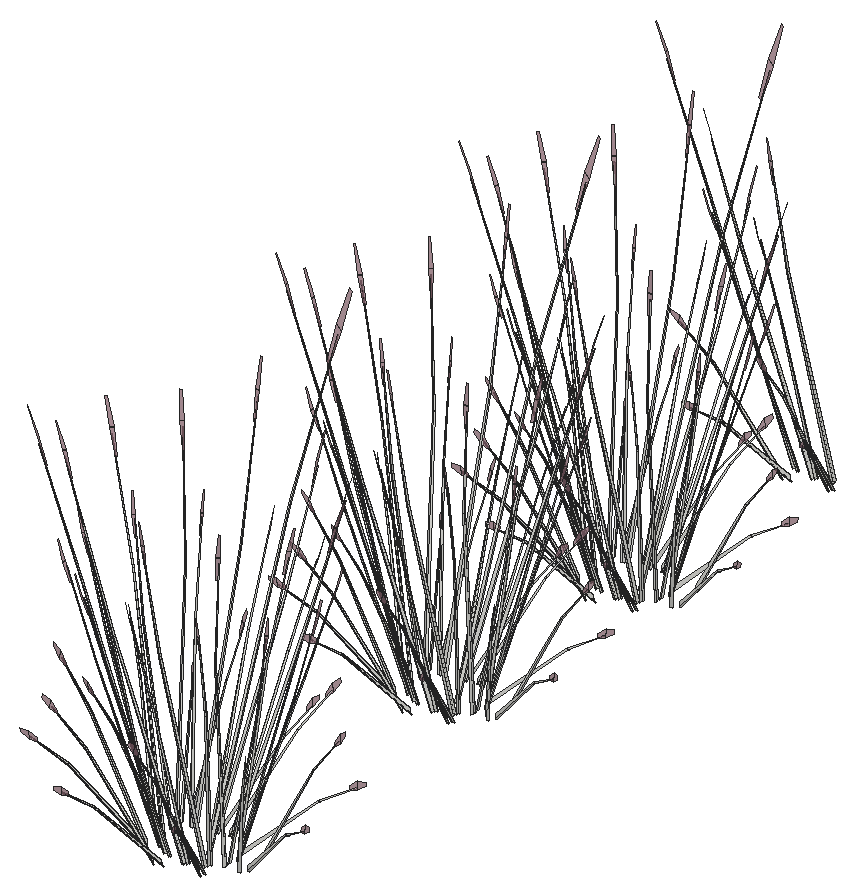
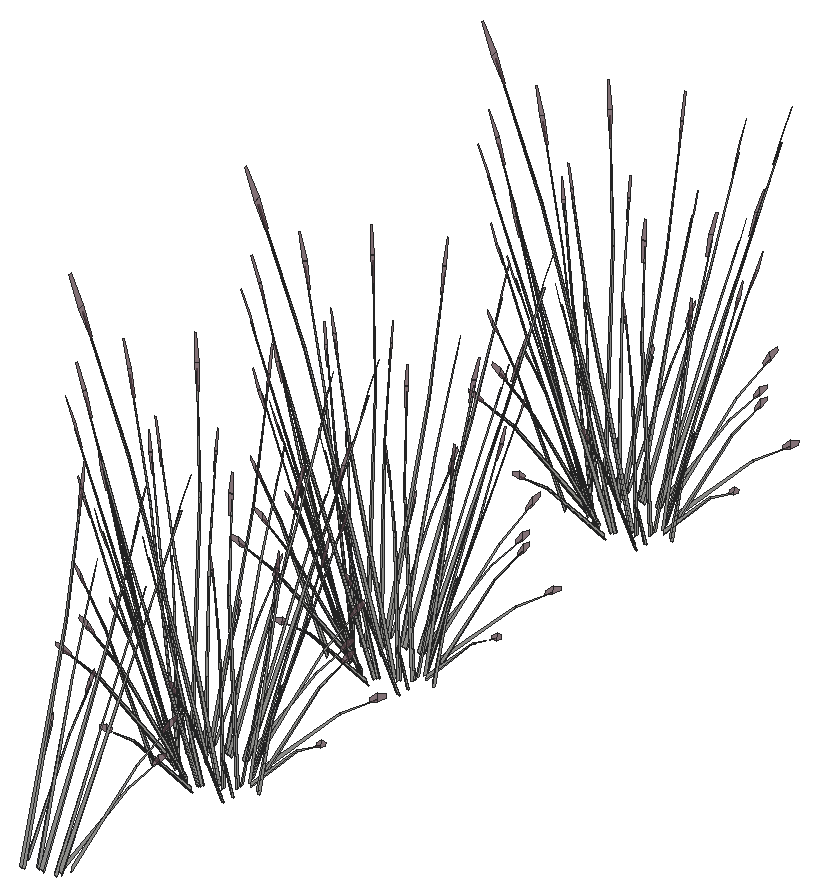
# SketchUp Ruby script. Lengths in inches.
U = 1.inch
M = Sketchup.active_model
def pt(a) = Geom::Point3d.new(a.map { |v| v * U })
def face(e, loops, mat)
  f = e.add_face(loops[0].map { |a| pt(a) })
  loops[1..].each { |l| e.add_face(l.map { |a| pt(a) }).erase! }
  f.material = f.back_material = mat if mat
  f
end
# faces: each face lists its corners as indices into pts; further lists are holes
def faces(e, pts, list, mat = nil) = list.each { |f| face(e, (f[0].is_a?(Array) ? f : [f]).map { |l| l.map { |i| pts[i] } }, mat) }
# xy, xz, yz: faces in a plane at the given z, y or x. An outline is a flat list of corners, or four numbers for a rectangle; further outlines are holes
def ring(l) = l.size == 4 ? [[l[0], l[1]], [l[2], l[1]], [l[2], l[3]], [l[0], l[3]]] : l.each_slice(2).to_a
def flat(e, list, mat, &to3) = list.each { |f| face(e, (f[0].is_a?(Array) ? f : [f]).map { |l| ring(l).map { |u, v| to3.(u, v) } }, mat) }
def xy(e, z, list, mat = nil) = flat(e, list, mat) { |x, y| [x, y, z] }
def xz(e, y, list, mat = nil) = flat(e, list, mat) { |x, z| [x, y, z] }
def yz(e, x, list, mat = nil) = flat(e, list, mat) { |y, z| [x, y, z] }
def lines(e, pts, list) = list.each { |a, b| e.add_line(pt(pts[a]), pt(pts[b])) }
# prism: a flat outline (further loops are holes) pulled along v
def prism(e, loops, v, mat = nil)
  f = face(e, loops, mat); d = Geom::Vector3d.new(v.map { |x| x * U })
  f.pushpull(f.normal.samedirection?(d) ? d.length : -d.length)
end
def box(e, o, s, mat = nil) = prism(e, [[o, [o[0] + s[0], o[1], o[2]], [o[0] + s[0], o[1] + s[1], o[2]], [o[0], o[1] + s[1], o[2]]]], [0, 0, s[2]], mat)
def at(x, y, z, deg = 0) = Geom::Transformation.translation(pt([x, y, z])) * Geom::Transformation.rotation(ORIGIN, Z_AXIS, deg.degrees)
def axes(o, x, y, z) = Geom::Transformation.new([*x, 0, *y, 0, *z, 0, *pt(o).to_a, 1])
def part(name) = M.definitions.add(name)
# library, detail: a bought-in or finely detailed component or shape, given as its bounding box
def library(name, o, s) = part(name).tap { |d| box(d.entities, o, s) }
def detail(e, o, s) = box(e.add_group.entities, o, s)
def put(e, d, t, mat = nil) = e.add_instance(d, t).tap { |i| i.material = mat if mat }
def group(e, t, mat = nil) = e.add_group.tap { |g| g.transformation = t; g.material = mat if mat }.entities
root = M.entities
M.materials.add("LightPink_Translucent").color = [144, 107, 117]
M.materials["LightPink_Translucent"].alpha = 0.75
c1 = part("blade")
p = [[2.15,0.21,22],[0,0.17,0],[0.09,0.45,0],[2.18,0.31,22],[2.29,0.31,22],[0.38,0.45,0],
  [2.48,0.24,33],[2.49,0.24,33],[2.48,0.22,33]]
faces(c1.entities,p,[[0,1,2,3],[4,5,2,3],[6,3,4,7],[8,0,3,6]])
c2 = part("seeds")
p = [[0.3,-0.1,1.38],[-0.01,-0.03,1.59],[-0.01,-0.03,0.03],[0.14,-0.07,-0.07],[0.29,-0.03,3],[0.15,0.01,3.11]]
faces(c2.entities,p,[[0,1,2,3],[1,0,4,5]],"LightPink_Translucent")
c3 = part("blade with seeds")
put(c3.entities,c1,at(0,0,0))
put(c3.entities,c2,axes([2.4,0.25,30.99],[1.5799,-0.05474,1.17369],[-0.12525,1.92788,0.29478],[-0.07173,-0.02425,1.56792]))
put(root,c3,axes([671.4,165.1,513.91],[-0.09951,-0.08005,1.45204],[-0.66407,0.05075,-0.22964],[-0.10598,-0.19148,0.11645]))
put(root,c3,axes([674.39,166.08,513.91],[-0.00628,-0.11364,1.45204],[-0.53042,-0.32843,-0.22964],[0.08201,-0.19909,0.11645]))
put(root,c3,axes([674.24,165.68,513.91],[-0.06607,0.04361,1.47228],[-0.64734,-0.14714,-0.13912],[-0.02343,-0.19032,0.26054]))
put(root,c3,axes([670.72,164.84,513.91],[-0.01214,0.06844,1.47228],[-0.59861,0.24837,-0.13912],[-0.17615,-0.12696,0.26054]))
put(root,c3,axes([672.41,166.34,514.18],[-0.63664,0.26583,-0.10093],[-0.31286,-0.47181,-0.56021],[-0.084,-0.19882,0.85122]))
put(root,c3,axes([673.74,166.9375,514.18],[-0.71502,-0.02829,-0.10093],[0.01954,-0.53563,-0.56021],[0.04967,-0.20629,0.85122]))
put(root,c3,axes([672.4,166.125,513.93],[0.47939,-0.19405,0.05337],[0.23464,0.35385,0.42015],[-0.0463,-0.15598,0.64067]))
put(root,c3,axes([670.76,166.18,513.93],[0.29569,-0.36271,0.05337],[0.42107,0.21117,0.42015],[-0.13613,-0.11629,0.64067]))
put(root,c3,axes([670.89,166.14,514.51],[-0.4342,0.54737,-0.11304],[-0.6288,-0.31535,-0.62743],[-0.21858,-0.15465,0.95337]))
put(root,c3,axes([673.85,166.75,513.93],[0.53464,0.0266,0.05337],[-0.01466,0.40172,0.42015],[0.05594,-0.15388,0.64067]))
put(root,c3,axes([669.22,165.98,513.91],[-0.13998,-0.00403,1.45204],[-0.44565,0.40302,-0.22964],[-0.23779,-0.08235,0.11645]))
put(root,c3,axes([674.51,167.99,514.18],[-0.60181,-0.31483,-0.10093],[0.34671,-0.45593,-0.56021],[0.17003,-0.15849,0.85122]))
put(root,c3,axes([675.99,167.85,513.91],[-0.08498,-0.00434,1.47228],[-0.35287,-0.46464,-0.13912],[0.14171,-0.15278,0.26054]))
put(root,c3,axes([669.37,166.89,513.93],[0.03276,-0.43418,0.05337],[0.49468,0.0119,0.42015],[-0.18949,-0.04543,0.64067]))
put(root,c3,axes([674.73,167.875,513.93],[0.44663,0.24013,0.05337],[-0.26003,0.34195,0.42015],[0.14319,-0.11055,0.64067]))
put(root,c3,axes([676.32,168.41,513.91],[0.09028,-0.08697,1.45204],[-0.11555,-0.53348,-0.22964],[0.22652,-0.10115,0.11645]))
put(root,c3,axes([668.6875,166.33,513.91],[0.04823,0.05698,1.47228],[-0.23252,0.51221,-0.13912],[-0.23548,0.00371,0.26054]))
put(root,c3,axes([669.6,166.99,514.18],[-0.03484,0.58066,-0.10093],[-0.65957,-0.01587,-0.56021],[-0.25402,-0.04034,0.85122]))
put(root,c3,axes([674.54,169.22,514.18],[-0.32734,-0.51701,-0.10093],[0.58097,-0.25407,-0.56021],[0.24483,-0.06821,0.85122]))
put(root,c3,axes([668.6,168.08,513.93],[-0.23895,-0.38931,0.05337],[0.43573,-0.19055,0.42015],[-0.19208,0.0376,0.64067]))
put(root,c3,axes([674.8,169.21,513.93],[0.23895,0.38931,0.05337],[-0.43573,0.19055,0.42015],[0.19208,-0.0376,0.64067]))
put(root,c3,axes([675.84,170.75,513.91],[-0.05883,-0.04999,1.47228],[0.12868,-0.53581,-0.13912],[0.23172,-0.03423,0.26054]))
put(root,c3,axes([668.18,168.58,513.91],[-0.10624,0.07413,1.45204],[0.00904,0.54162,-0.22964],[-0.24352,0.07044,0.11645]))
put(root,c3,axes([668.87,168.0625,514.18],[0.32734,0.51701,-0.10093],[-0.58097,0.25407,-0.56021],[-0.24483,0.06821,0.85122]))
put(root,c3,axes([673.8,170.29,514.18],[0.03484,-0.58066,-0.10093],[0.65957,0.01587,-0.56021],[0.25402,0.04034,0.85122]))
put(root,c3,axes([674.375,169.94,513.91],[0.13956,-0.00966,1.45204],[0.38281,-0.44358,-0.22964],[0.24825,0.05855,0.11645]))
put(root,c3,axes([668.67,169.41,513.93],[-0.44663,-0.24013,0.05337],[0.26003,-0.34195,0.42015],[-0.14319,0.11055,0.64067]))
put(root,c3,axes([667,169.13,513.91],[0.08303,0.01531,1.47228],[0.25685,0.50448,-0.13912],[-0.16996,0.13241,0.26054]))
put(root,c3,axes([674.04,170.39,513.93],[-0.03276,0.43418,0.05337],[-0.49468,-0.0119,0.42015],[0.18949,0.04543,0.64067]))
put(root,c3,axes([672.94,168.04,513.71],[-0.56218,-0.29666,1.14775],[0.59361,-0.46189,0.49522],[0.18138,0.27836,1.10941]))
put(root,c3,axes([668.89,169.29,514.18],[0.60181,0.31483,-0.10093],[-0.34671,0.45593,-0.56021],[-0.17003,0.15849,0.85122]))
put(root,c3,axes([672.5,170.92,514.18],[0.38768,-0.48872,-0.10093],[0.56143,0.28156,-0.56021],[0.19516,0.13808,0.85122]))
put(root,c3,axes([672,171.33,513.91],[0.00193,-0.06913,1.47228],[0.55753,-0.30498,-0.13912],[0.19366,0.10886,0.26054]))
put(root,c3,axes([669.55,170.54,513.93],[-0.53464,-0.0266,0.05337],[0.01466,-0.40172,0.42015],[-0.05594,0.15388,0.64067]))
put(root,c3,axes([672.65,171.1,513.93],[-0.29569,0.36271,0.05337],[-0.42107,-0.21117,0.42015],[0.13613,0.11629,0.64067]))
put(root,c3,axes([671,171.16,513.93],[-0.47939,0.19405,0.05337],[-0.23464,-0.35385,0.42015],[0.0463,0.15598,0.64067]))
put(root,c3,axes([668.2,170.6,513.91],[-0.01617,0.11299,1.45204],[0.45894,0.39307,-0.22964],[-0.12015,0.18588,0.11645]))
put(root,c3,axes([669.67,170.35,514.48],[0.71502,0.02829,-0.11203],[-0.01954,0.53563,-0.62183],[-0.04967,0.20629,0.94486]))
put(root,c3,axes([670.99,170.94,514.18],[0.63664,-0.26583,-0.10093],[0.31286,0.47181,-0.56021],[0.084,0.19882,0.85122]))
put(root,c3,axes([668.15,171.76,513.91],[0.07381,-0.03447,1.47228],[0.61004,0.22929,-0.13912],[-0.01434,0.19091,0.26054]))
put(root,c3,axes([670.84,172,513.91],[0.08247,0.09194,1.45204],[0.66552,0.03612,-0.22964],[0.06692,0.20277,0.11645]))
put(root,c3,axes([671.4,192.5625,513.91],[-0.09951,-0.08005,1.45204],[-0.66407,0.05075,-0.22964],[-0.10598,-0.19148,0.11645]))
put(root,c3,axes([674.39,193.54,513.91],[-0.00628,-0.11364,1.45204],[-0.53042,-0.32843,-0.22964],[0.08201,-0.19909,0.11645]))
put(root,c3,axes([674.24,193.13,513.91],[-0.06607,0.04361,1.47228],[-0.64734,-0.14714,-0.13912],[-0.02343,-0.19032,0.26054]))
put(root,c3,axes([670.72,192.3,513.91],[-0.01214,0.06844,1.47228],[-0.59861,0.24837,-0.13912],[-0.17615,-0.12696,0.26054]))
put(root,c3,axes([672.41,193.8,514.18],[-0.63664,0.26583,-0.10093],[-0.31286,-0.47181,-0.56021],[-0.084,-0.19882,0.85122]))
put(root,c3,axes([673.74,194.39,514.18],[-0.71502,-0.02829,-0.10093],[0.01954,-0.53563,-0.56021],[0.04967,-0.20629,0.85122]))
put(root,c3,axes([672.4,193.58,513.93],[0.47939,-0.19405,0.05337],[0.23464,0.35385,0.42015],[-0.0463,-0.15598,0.64067]))
put(root,c3,axes([670.76,193.64,513.93],[0.29569,-0.36271,0.05337],[0.42107,0.21117,0.42015],[-0.13613,-0.11629,0.64067]))
put(root,c3,axes([670.89,193.6,514.51],[-0.4342,0.54737,-0.11304],[-0.6288,-0.31535,-0.62743],[-0.21858,-0.15465,0.95337]))
put(root,c3,axes([673.85,194.2,513.93],[0.53464,0.0266,0.05337],[-0.01466,0.40172,0.42015],[0.05594,-0.15388,0.64067]))
put(root,c3,axes([669.22,193.44,513.91],[-0.13998,-0.00403,1.45204],[-0.44565,0.40302,-0.22964],[-0.23779,-0.08235,0.11645]))
put(root,c3,axes([674.51,195.45,514.18],[-0.60181,-0.31483,-0.10093],[0.34671,-0.45593,-0.56021],[0.17003,-0.15849,0.85122]))
put(root,c3,axes([675.99,195.3125,513.91],[-0.08498,-0.00434,1.47228],[-0.35287,-0.46464,-0.13912],[0.14171,-0.15278,0.26054]))
put(root,c3,axes([669.37,194.35,513.93],[0.03276,-0.43418,0.05337],[0.49468,0.0119,0.42015],[-0.18949,-0.04543,0.64067]))
put(root,c3,axes([674.73,195.33,513.93],[0.44663,0.24013,0.05337],[-0.26003,0.34195,0.42015],[0.14319,-0.11055,0.64067]))
put(root,c3,axes([676.32,195.87,513.91],[0.09028,-0.08697,1.45204],[-0.11555,-0.53348,-0.22964],[0.22652,-0.10115,0.11645]))
put(root,c3,axes([668.6875,193.78,513.91],[0.04823,0.05698,1.47228],[-0.23252,0.51221,-0.13912],[-0.23548,0.00371,0.26054]))
put(root,c3,axes([669.6,194.45,514.18],[-0.03484,0.58066,-0.10093],[-0.65957,-0.01587,-0.56021],[-0.25402,-0.04034,0.85122]))
put(root,c3,axes([674.54,196.68,514.18],[-0.32734,-0.51701,-0.10093],[0.58097,-0.25407,-0.56021],[0.24483,-0.06821,0.85122]))
put(root,c3,axes([668.6,195.53,513.93],[-0.23895,-0.38931,0.05337],[0.43573,-0.19055,0.42015],[-0.19208,0.0376,0.64067]))
put(root,c3,axes([674.8,196.66,513.93],[0.23895,0.38931,0.05337],[-0.43573,0.19055,0.42015],[0.19208,-0.0376,0.64067]))
put(root,c3,axes([675.84,198.21,513.91],[-0.05883,-0.04999,1.47228],[0.12868,-0.53581,-0.13912],[0.23172,-0.03423,0.26054]))
put(root,c3,axes([668.18,196.04,513.91],[-0.10624,0.07413,1.45204],[0.00904,0.54162,-0.22964],[-0.24352,0.07044,0.11645]))
put(root,c3,axes([668.87,195.52,514.18],[0.32734,0.51701,-0.10093],[-0.58097,0.25407,-0.56021],[-0.24483,0.06821,0.85122]))
put(root,c3,axes([673.8,197.75,514.18],[0.03484,-0.58066,-0.10093],[0.65957,0.01587,-0.56021],[0.25402,0.04034,0.85122]))
put(root,c3,axes([674.375,197.4,513.91],[0.13956,-0.00966,1.45204],[0.38281,-0.44358,-0.22964],[0.24825,0.05855,0.11645]))
put(root,c3,axes([668.67,196.87,513.93],[-0.44663,-0.24013,0.05337],[0.26003,-0.34195,0.42015],[-0.14319,0.11055,0.64067]))
put(root,c3,axes([667,196.59,513.91],[0.08303,0.01531,1.47228],[0.25685,0.50448,-0.13912],[-0.16996,0.13241,0.26054]))
put(root,c3,axes([674.04,197.85,513.93],[-0.03276,0.43418,0.05337],[-0.49468,-0.0119,0.42015],[0.18949,0.04543,0.64067]))
put(root,c3,axes([672.94,195.5,513.71],[-0.56218,-0.29666,1.14775],[0.59361,-0.46189,0.49522],[0.18138,0.27836,1.10941]))
put(root,c3,axes([668.89,196.75,514.18],[0.60181,0.31483,-0.10093],[-0.34671,0.45593,-0.56021],[-0.17003,0.15849,0.85122]))
put(root,c3,axes([672.5,198.38,514.18],[0.38768,-0.48872,-0.10093],[0.56143,0.28156,-0.56021],[0.19516,0.13808,0.85122]))
put(root,c3,axes([672,198.79,513.91],[0.00193,-0.06913,1.47228],[0.55753,-0.30498,-0.13912],[0.19366,0.10886,0.26054]))
put(root,c3,axes([669.55,197.99,513.93],[-0.53464,-0.0266,0.05337],[0.01466,-0.40172,0.42015],[-0.05594,0.15388,0.64067]))
put(root,c3,axes([672.65,198.5625,513.93],[-0.29569,0.36271,0.05337],[-0.42107,-0.21117,0.42015],[0.13613,0.11629,0.64067]))
put(root,c3,axes([671,198.61,513.93],[-0.47939,0.19405,0.05337],[-0.23464,-0.35385,0.42015],[0.0463,0.15598,0.64067]))
put(root,c3,axes([668.2,198.06,513.91],[-0.01617,0.11299,1.45204],[0.45894,0.39307,-0.22964],[-0.12015,0.18588,0.11645]))
put(root,c3,axes([669.67,197.8,514.48],[0.71502,0.02829,-0.11203],[-0.01954,0.53563,-0.62183],[-0.04967,0.20629,0.94486]))
put(root,c3,axes([670.99,198.4,514.18],[0.63664,-0.26583,-0.10093],[0.31286,0.47181,-0.56021],[0.084,0.19882,0.85122]))
put(root,c3,axes([668.15,199.22,513.91],[0.07381,-0.03447,1.47228],[0.61004,0.22929,-0.13912],[-0.01434,0.19091,0.26054]))
put(root,c3,axes([670.84,199.46,513.91],[0.08247,0.09194,1.45204],[0.66552,0.03612,-0.22964],[0.06692,0.20277,0.11645]))
put(root,c3,axes([671.4,212.85,513.91],[-0.09951,-0.08005,1.45204],[-0.66407,0.05075,-0.22964],[-0.10598,-0.19148,0.11645]))
put(root,c3,axes([674.39,213.83,513.91],[-0.00628,-0.11364,1.45204],[-0.53042,-0.32843,-0.22964],[0.08201,-0.19909,0.11645]))
put(root,c3,axes([674.24,213.43,513.91],[-0.06607,0.04361,1.47228],[-0.64734,-0.14714,-0.13912],[-0.02343,-0.19032,0.26054]))
put(root,c3,axes([670.72,212.59,513.91],[-0.01214,0.06844,1.47228],[-0.59861,0.24837,-0.13912],[-0.17615,-0.12696,0.26054]))
put(root,c3,axes([672.41,214.09,514.18],[-0.63664,0.26583,-0.10093],[-0.31286,-0.47181,-0.56021],[-0.084,-0.19882,0.85122]))
put(root,c3,axes([673.74,214.69,514.18],[-0.71502,-0.02829,-0.10093],[0.01954,-0.53563,-0.56021],[0.04967,-0.20629,0.85122]))
put(root,c3,axes([672.4,213.875,513.93],[0.47939,-0.19405,0.05337],[0.23464,0.35385,0.42015],[-0.0463,-0.15598,0.64067]))
put(root,c3,axes([670.76,213.93,513.93],[0.29569,-0.36271,0.05337],[0.42107,0.21117,0.42015],[-0.13613,-0.11629,0.64067]))
put(root,c3,axes([670.89,213.89,514.51],[-0.4342,0.54737,-0.11304],[-0.6288,-0.31535,-0.62743],[-0.21858,-0.15465,0.95337]))
put(root,c3,axes([673.85,214.49,513.93],[0.53464,0.0266,0.05337],[-0.01466,0.40172,0.42015],[0.05594,-0.15388,0.64067]))
put(root,c3,axes([669.22,213.73,513.91],[-0.13998,-0.00403,1.45204],[-0.44565,0.40302,-0.22964],[-0.23779,-0.08235,0.11645]))
put(root,c3,axes([674.51,215.74,514.18],[-0.60181,-0.31483,-0.10093],[0.34671,-0.45593,-0.56021],[0.17003,-0.15849,0.85122]))
put(root,c3,axes([675.99,215.6,513.91],[-0.08498,-0.00434,1.47228],[-0.35287,-0.46464,-0.13912],[0.14171,-0.15278,0.26054]))
put(root,c3,axes([669.37,214.64,513.93],[0.03276,-0.43418,0.05337],[0.49468,0.0119,0.42015],[-0.18949,-0.04543,0.64067]))
put(root,c3,axes([674.73,215.62,513.93],[0.44663,0.24013,0.05337],[-0.26003,0.34195,0.42015],[0.14319,-0.11055,0.64067]))
put(root,c3,axes([676.32,216.16,513.91],[0.09028,-0.08697,1.45204],[-0.11555,-0.53348,-0.22964],[0.22652,-0.10115,0.11645]))
put(root,c3,axes([668.6875,214.08,513.91],[0.04823,0.05698,1.47228],[-0.23252,0.51221,-0.13912],[-0.23548,0.00371,0.26054]))
put(root,c3,axes([669.6,214.74,514.18],[-0.03484,0.58066,-0.10093],[-0.65957,-0.01587,-0.56021],[-0.25402,-0.04034,0.85122]))
put(root,c3,axes([674.54,216.97,514.18],[-0.32734,-0.51701,-0.10093],[0.58097,-0.25407,-0.56021],[0.24483,-0.06821,0.85122]))
put(root,c3,axes([668.6,215.83,513.93],[-0.23895,-0.38931,0.05337],[0.43573,-0.19055,0.42015],[-0.19208,0.0376,0.64067]))
put(root,c3,axes([674.8,216.96,513.93],[0.23895,0.38931,0.05337],[-0.43573,0.19055,0.42015],[0.19208,-0.0376,0.64067]))
put(root,c3,axes([675.84,218.5,513.91],[-0.05883,-0.04999,1.47228],[0.12868,-0.53581,-0.13912],[0.23172,-0.03423,0.26054]))
put(root,c3,axes([668.18,216.33,513.91],[-0.10624,0.07413,1.45204],[0.00904,0.54162,-0.22964],[-0.24352,0.07044,0.11645]))
put(root,c3,axes([668.87,215.8125,514.18],[0.32734,0.51701,-0.10093],[-0.58097,0.25407,-0.56021],[-0.24483,0.06821,0.85122]))
put(root,c3,axes([673.8,218.04,514.18],[0.03484,-0.58066,-0.10093],[0.65957,0.01587,-0.56021],[0.25402,0.04034,0.85122]))
put(root,c3,axes([674.375,217.69,513.91],[0.13956,-0.00966,1.45204],[0.38281,-0.44358,-0.22964],[0.24825,0.05855,0.11645]))
put(root,c3,axes([668.67,217.16,513.93],[-0.44663,-0.24013,0.05337],[0.26003,-0.34195,0.42015],[-0.14319,0.11055,0.64067]))
put(root,c3,axes([667,216.88,513.91],[0.08303,0.01531,1.47228],[0.25685,0.50448,-0.13912],[-0.16996,0.13241,0.26054]))
put(root,c3,axes([674.04,218.14,513.93],[-0.03276,0.43418,0.05337],[-0.49468,-0.0119,0.42015],[0.18949,0.04543,0.64067]))
put(root,c3,axes([672.94,215.79,513.71],[-0.56218,-0.29666,1.14775],[0.59361,-0.46189,0.49522],[0.18138,0.27836,1.10941]))
put(root,c3,axes([668.89,217.04,514.18],[0.60181,0.31483,-0.10093],[-0.34671,0.45593,-0.56021],[-0.17003,0.15849,0.85122]))
put(root,c3,axes([672.5,218.67,514.18],[0.38768,-0.48872,-0.10093],[0.56143,0.28156,-0.56021],[0.19516,0.13808,0.85122]))
put(root,c3,axes([672,219.08,513.91],[0.00193,-0.06913,1.47228],[0.55753,-0.30498,-0.13912],[0.19366,0.10886,0.26054]))
put(root,c3,axes([669.55,218.29,513.93],[-0.53464,-0.0266,0.05337],[0.01466,-0.40172,0.42015],[-0.05594,0.15388,0.64067]))
put(root,c3,axes([672.65,218.85,513.93],[-0.29569,0.36271,0.05337],[-0.42107,-0.21117,0.42015],[0.13613,0.11629,0.64067]))
put(root,c3,axes([671,218.91,513.93],[-0.47939,0.19405,0.05337],[-0.23464,-0.35385,0.42015],[0.0463,0.15598,0.64067]))
put(root,c3,axes([668.2,218.35,513.91],[-0.01617,0.11299,1.45204],[0.45894,0.39307,-0.22964],[-0.12015,0.18588,0.11645]))
put(root,c3,axes([669.67,218.1,514.48],[0.71502,0.02829,-0.11203],[-0.01954,0.53563,-0.62183],[-0.04967,0.20629,0.94486]))
put(root,c3,axes([670.99,218.69,514.18],[0.63664,-0.26583,-0.10093],[0.31286,0.47181,-0.56021],[0.084,0.19882,0.85122]))
put(root,c3,axes([668.15,219.51,513.91],[0.07381,-0.03447,1.47228],[0.61004,0.22929,-0.13912],[-0.01434,0.19091,0.26054]))
put(root,c3,axes([670.84,219.75,513.91],[0.08247,0.09194,1.45204],[0.66552,0.03612,-0.22964],[0.06692,0.20277,0.11645]))
put(root,c3,axes([671.4,234.55,513.91],[-0.09951,-0.08005,1.45204],[-0.66407,0.05075,-0.22964],[-0.10598,-0.19148,0.11645]))
put(root,c3,axes([674.39,235.53,513.91],[-0.00628,-0.11364,1.45204],[-0.53042,-0.32843,-0.22964],[0.08201,-0.19909,0.11645]))
put(root,c3,axes([674.24,235.125,513.91],[-0.06607,0.04361,1.47228],[-0.64734,-0.14714,-0.13912],[-0.02343,-0.19032,0.26054]))
put(root,c3,axes([670.72,234.29,513.91],[-0.01214,0.06844,1.47228],[-0.59861,0.24837,-0.13912],[-0.17615,-0.12696,0.26054]))
put(root,c3,axes([672.41,235.79,514.18],[-0.63664,0.26583,-0.10093],[-0.31286,-0.47181,-0.56021],[-0.084,-0.19882,0.85122]))
put(root,c3,axes([673.74,236.38,514.18],[-0.71502,-0.02829,-0.10093],[0.01954,-0.53563,-0.56021],[0.04967,-0.20629,0.85122]))
put(root,c3,axes([672.4,235.57,513.93],[0.47939,-0.19405,0.05337],[0.23464,0.35385,0.42015],[-0.0463,-0.15598,0.64067]))
put(root,c3,axes([670.76,235.625,513.93],[0.29569,-0.36271,0.05337],[0.42107,0.21117,0.42015],[-0.13613,-0.11629,0.64067]))
put(root,c3,axes([670.89,235.59,514.51],[-0.4342,0.54737,-0.11304],[-0.6288,-0.31535,-0.62743],[-0.21858,-0.15465,0.95337]))
